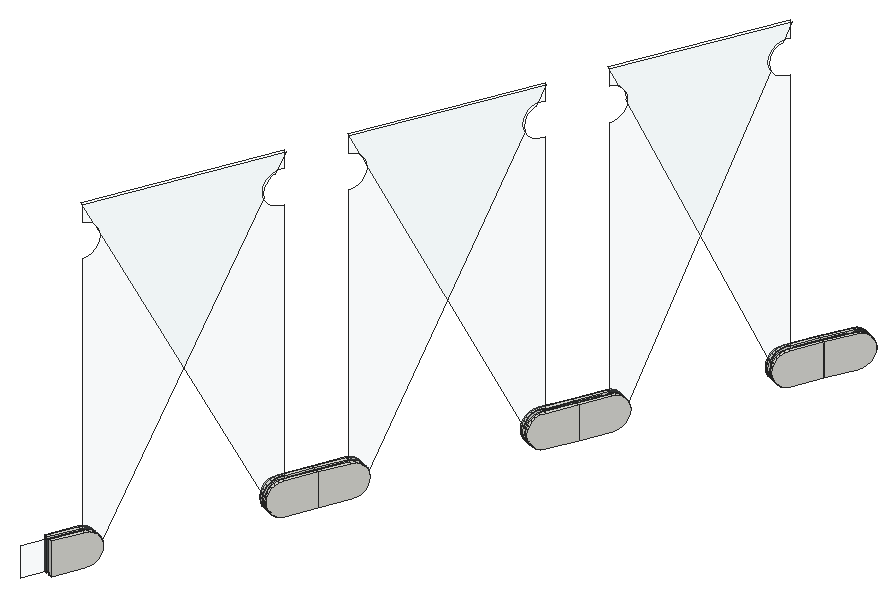
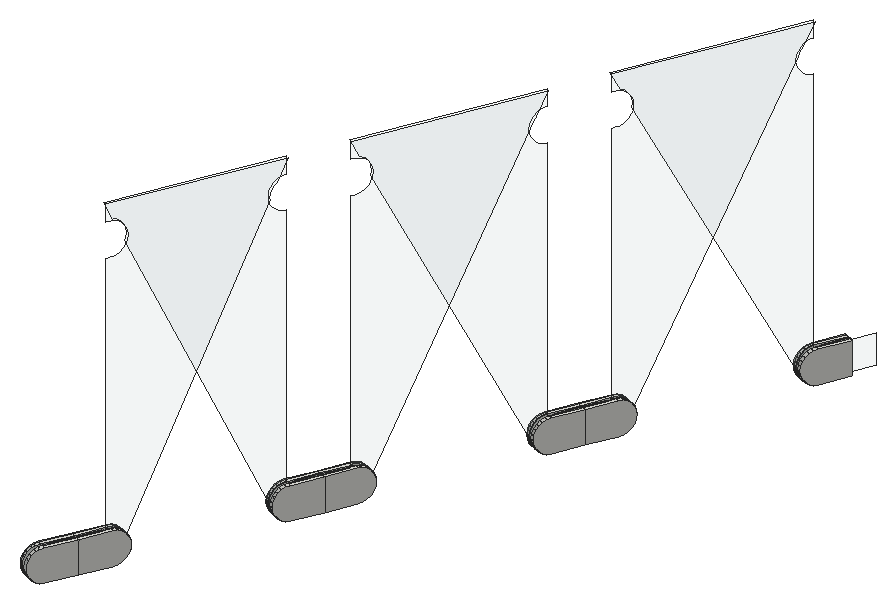
# SketchUp Ruby script. Lengths in inches.
U = 1.inch
M = Sketchup.active_model
def pt(a) = Geom::Point3d.new(a.map { |v| v * U })
def face(e, loops, mat)
  f = e.add_face(loops[0].map { |a| pt(a) })
  loops[1..].each { |l| e.add_face(l.map { |a| pt(a) }).erase! }
  f.material = f.back_material = mat if mat
  f
end
# faces: each face lists its corners as indices into pts; further lists are holes
def faces(e, pts, list, mat = nil) = list.each { |f| face(e, (f[0].is_a?(Array) ? f : [f]).map { |l| l.map { |i| pts[i] } }, mat) }
# xy, xz, yz: faces in a plane at the given z, y or x. An outline is a flat list of corners, or four numbers for a rectangle; further outlines are holes
def ring(l) = l.size == 4 ? [[l[0], l[1]], [l[2], l[1]], [l[2], l[3]], [l[0], l[3]]] : l.each_slice(2).to_a
def flat(e, list, mat, &to3) = list.each { |f| face(e, (f[0].is_a?(Array) ? f : [f]).map { |l| ring(l).map { |u, v| to3.(u, v) } }, mat) }
def xy(e, z, list, mat = nil) = flat(e, list, mat) { |x, y| [x, y, z] }
def xz(e, y, list, mat = nil) = flat(e, list, mat) { |x, z| [x, y, z] }
def yz(e, x, list, mat = nil) = flat(e, list, mat) { |y, z| [x, y, z] }
def lines(e, pts, list) = list.each { |a, b| e.add_line(pt(pts[a]), pt(pts[b])) }
# prism: a flat outline (further loops are holes) pulled along v
def prism(e, loops, v, mat = nil)
  f = face(e, loops, mat); d = Geom::Vector3d.new(v.map { |x| x * U })
  f.pushpull(f.normal.samedirection?(d) ? d.length : -d.length)
end
def box(e, o, s, mat = nil) = prism(e, [[o, [o[0] + s[0], o[1], o[2]], [o[0] + s[0], o[1] + s[1], o[2]], [o[0], o[1] + s[1], o[2]]]], [0, 0, s[2]], mat)
def at(x, y, z, deg = 0) = Geom::Transformation.translation(pt([x, y, z])) * Geom::Transformation.rotation(ORIGIN, Z_AXIS, deg.degrees)
def axes(o, x, y, z) = Geom::Transformation.new([*x, 0, *y, 0, *z, 0, *pt(o).to_a, 1])
def part(name) = M.definitions.add(name)
# library, detail: a bought-in or finely detailed component or shape, given as its bounding box
def library(name, o, s) = part(name).tap { |d| box(d.entities, o, s) }
def detail(e, o, s) = box(e.add_group.entities, o, s)
def put(e, d, t, mat = nil) = e.add_instance(d, t).tap { |i| i.material = mat if mat }
def group(e, t, mat = nil) = e.add_group.tap { |g| g.transformation = t; g.material = mat if mat }.entities
root = M.entities
M.materials.add("Glass_Safety_01").color = [204, 235, 244]
M.materials["Glass_Safety_01"].alpha = 0.1
xy(root,333,[[858.978,571.145,858.726,571.255,859.512,573.06,859.764,572.949],[858.545,571.333,858.292,571.443,859.078,573.248,859.331,573.138],[864.446,583.7,864.194,583.81,864.292,584.037,864.98,585.615,865.232,585.505],[864.013,583.889,863.761,583.999,864.547,585.803,864.799,585.693,864.112,584.115],[865.232,585.505,864.98,585.615,865.766,587.42,866.018,587.309],
  [864.799,585.693,864.547,585.803,865.333,587.608,865.585,587.498],[870.556,597.727,870.303,597.837,870.404,598.069,871.089,599.642,871.341,599.53],[870.122,597.916,869.87,598.026,870.656,599.83,870.908,599.72,870.224,598.148],[871.341,599.53,871.089,599.642,871.342,599.532],[871.342,599.532,871.089,599.642,871.885,601.441,872.137,601.33],
  [870.908,599.72,870.656,599.832,871.453,601.633,871.705,601.521],[876.349,610.851,876.097,610.963,876.207,611.21,876.893,612.761,877.142,612.643],[875.917,611.043,875.665,611.154,876.462,612.954,876.714,612.843,876.027,611.29],[877.142,612.643,876.893,612.761,876.894,612.763,877.146,612.652,877.144,612.647],[877.146,612.652,876.894,612.763,877.734,614.541,877.983,614.423],
  [876.715,612.845,876.466,612.963,877.307,614.743,877.556,614.625]])
xy(root,333.078,[[858.726,571.255,858.545,571.333,859.174,572.777,859.354,572.699],[864.351,584.171,864.17,584.25,864.799,585.693,864.98,585.615],[864.98,585.615,864.799,585.693,865.428,587.137,865.609,587.059],[870.46,598.198,870.28,598.277,870.908,599.72,870.999,599.681,871.089,599.642],[871.089,599.642,870.999,599.681,870.908,599.72,871.546,601.161,871.726,601.081],
  [876.257,611.323,876.077,611.403,876.714,612.843,876.804,612.803,876.893,612.761],[876.893,612.761,876.804,612.803,876.894,612.763,876.893,612.762],[876.894,612.763,876.804,612.803,876.715,612.845,877.388,614.269,877.566,614.185]],"Glass_Safety_01")
xy(root,335.047,[[858.726,571.255,859.354,572.699,859.174,572.777,858.545,571.333],[864.351,584.171,864.98,585.615,864.799,585.693,864.17,584.25],[864.98,585.615,865.609,587.059,865.428,587.137,864.799,585.693],[870.46,598.198,871.089,599.642,870.999,599.681,870.908,599.72,870.28,598.277],[871.089,599.642,871.726,601.081,871.546,601.161,870.908,599.72,870.999,599.681],
  [876.257,611.323,876.893,612.761,876.804,612.803,876.714,612.843,876.077,611.403],[876.893,612.761,876.893,612.762,876.894,612.763,876.804,612.803],[876.894,612.763,877.566,614.185,877.388,614.269,876.715,612.845,876.804,612.803]],"Glass_Safety_01")
xy(root,335.126,[[858.978,571.145,859.764,572.949,859.512,573.06,858.726,571.255],[858.545,571.333,859.331,573.138,859.078,573.248,858.292,571.443],[864.446,583.7,865.232,585.505,864.98,585.615,864.292,584.037,864.194,583.81],[864.013,583.889,864.112,584.115,864.799,585.693,864.547,585.803,863.761,583.999],[865.232,585.505,866.018,587.309,865.766,587.42,864.98,585.615],
  [864.799,585.693,865.585,587.498,865.333,587.608,864.547,585.803],[870.556,597.727,871.341,599.53,871.089,599.642,870.404,598.069,870.303,597.837],[870.122,597.916,870.224,598.148,870.908,599.72,870.656,599.83,869.87,598.026],[871.341,599.53,871.342,599.532,871.089,599.642],[871.342,599.532,872.137,601.33,871.885,601.441,871.089,599.642],
  [870.908,599.72,871.705,601.521,871.453,601.633,870.656,599.832],[876.349,610.851,877.142,612.643,876.893,612.761,876.207,611.21,876.097,610.963],[875.917,611.043,876.027,611.29,876.714,612.843,876.462,612.954,875.665,611.154],[877.142,612.643,877.144,612.647,877.146,612.652,876.894,612.763,876.893,612.761],[877.146,612.652,877.983,614.423,877.734,614.541,876.894,612.763],
  [876.715,612.845,877.556,614.625,877.307,614.743,876.466,612.963]])
p = [[858.726,571.255,333],[858.726,571.255,333.078],[858.726,571.255,335.047],[858.726,571.255,335.126],[858.978,571.145,335.126],[858.978,571.145,333],
  [859.764,572.949,335.126],[859.764,572.949,333],[859.874,573.202,333.036],[859.976,573.437,333.142],[860.064,573.639,333.311],[860.132,573.793,333.531],
  [860.174,573.891,333.787],[860.189,573.924,334.0625],[860.174,573.891,334.338],[860.132,573.793,334.594],[860.064,573.639,334.814],[859.976,573.437,334.983],
  [859.874,573.202,335.089],[858.545,571.333,333.078],[858.545,571.333,333],[858.292,571.443,333],[858.292,571.443,335.126],[858.545,571.333,335.126],
  [858.545,571.333,335.047],[859.331,573.138,333],[859.331,573.138,335.126],[859.174,572.777,335.047],[859.174,572.777,333.078],[859.512,573.06,335.126],
  [859.512,573.06,333],[859.354,572.699,333.078],[859.354,572.699,335.047],[859.078,573.248,335.126],[859.188,573.5,335.089],[859.291,573.735,334.983],
  [859.379,573.9375,334.814],[859.446,574.092,334.594],[859.488,574.19,334.338],[859.503,574.223,334.0625],[859.488,574.19,333.787],[859.446,574.092,333.531],
  [859.379,573.9375,333.311],[859.291,573.735,333.142],[859.188,573.5,333.036],[859.078,573.248,333],[859.621,573.312,333.036],[859.441,573.39,333.036],
  [859.441,573.39,335.089],[859.543,573.625,334.983],[859.631,573.827,334.814],[859.699,573.982,334.594],[859.741,574.08,334.338],[859.756,574.113,334.0625],
  [859.741,574.08,333.787],[859.699,573.982,333.531],[859.631,573.827,333.311],[859.543,573.625,333.142],[859.925,574.009,333.853],[859.81,573.744,333.307],
  [859.724,573.547,333.142],[859.621,573.312,335.089],[859.724,573.547,334.983],[859.812,573.749,334.814],[859.879,573.904,334.594],[859.922,574.001,334.338],
  [859.936,574.034,334.0625],[865.232,585.505,335.126],[864.446,583.7,335.126],[864.337,583.448,335.089],[864.234,583.213,334.983],[864.146,583.011,334.814],
  [864.079,582.856,334.594],[864.036,582.759,334.338],[864.022,582.725,334.0625],[864.036,582.759,333.787],[864.079,582.856,333.531],[864.146,583.011,333.311],
  [864.234,583.213,333.142],[864.337,583.448,333.036],[864.446,583.7,333],[865.232,585.505,333],[864.194,583.81,335.126],[864.292,584.037,335.126],
  [864.292,584.037,333],[864.194,583.81,333],[864.084,583.558,333.036],[863.981,583.323,333.142],[863.894,583.121,333.311],[863.826,582.966,333.531],
  [863.784,582.869,333.787],[863.769,582.835,334.0625],[863.784,582.869,334.338],[863.826,582.966,334.594],[863.894,583.121,334.814],[863.981,583.323,334.983],
  [864.084,583.558,335.089],[863.602,582.944,334.311],[863.862,583.542,333.078],[863.903,583.636,333.036],[864.013,583.889,333],[864.112,584.115,333],
  [864.112,584.115,335.126],[864.013,583.889,335.126],[863.903,583.636,335.089],[863.801,583.401,334.983],[863.713,583.199,334.814],[863.646,583.045,334.594],
  [863.603,582.947,334.338],[863.761,583.999,335.126],[864.547,585.803,335.126],[864.547,585.803,333],[863.761,583.999,333],[863.651,583.746,333.036],
  [863.548,583.511,333.142],[863.46,583.31,333.311],[863.393,583.155,333.531],[863.351,583.057,333.787],[863.336,583.024,334.0625],[863.351,583.057,334.338],
  [863.393,583.155,334.594],[863.46,583.31,334.814],[863.548,583.511,334.983],[863.651,583.746,335.089],[863.801,583.401,333.142],[864.98,585.615,333],
  [864.98,585.615,335.126],[864.98,585.615,335.047],[864.351,584.171,335.047],[864.351,584.171,333.078],[864.98,585.615,333.078],[864.799,585.693,335.126],
  [864.799,585.693,333],[864.799,585.693,333.078],[864.17,584.25,333.078],[864.17,584.25,335.047],[864.799,585.693,335.047],[866.018,587.309,335.126],
  [866.018,587.309,333],[866.128,587.562,333.036],[866.231,587.797,333.142],[866.319,587.999,333.311],[866.386,588.153,333.531],[866.428,588.251,333.787],
  [866.443,588.284,334.0625],[866.428,588.251,334.338],[866.386,588.153,334.594],[866.319,587.999,334.814],[866.231,587.797,334.983],[866.128,587.562,335.089],
  [865.766,587.42,335.126],[865.766,587.42,333],[865.609,587.059,333.078],[865.609,587.059,335.047],[865.585,587.498,333],[865.585,587.498,335.126],
  [865.428,587.137,335.047],[865.428,587.137,333.078],[865.333,587.608,335.126],[865.442,587.86,335.089],[865.545,588.095,334.983],[865.633,588.297,334.814],
  [865.7,588.452,334.594],[865.743,588.55,334.338],[865.757,588.583,334.0625],[865.743,588.55,333.787],[865.7,588.452,333.531],[865.633,588.297,333.311],
  [865.545,588.095,333.142],[865.442,587.86,333.036],[865.333,587.608,333],[865.876,587.672,333.036],[866.183,588.379,333.934],[866.049,588.07,333.279],
  [865.978,587.907,333.142],[865.876,587.672,335.089],[865.978,587.907,334.983],[866.066,588.109,334.814],[866.133,588.264,334.594],[866.176,588.361,334.338],
  [866.19,588.394,334.0625],[865.695,587.75,333.036],[865.695,587.75,335.089],[865.798,587.985,334.983],[865.885,588.187,334.814],[865.953,588.342,334.594],
  [865.995,588.439,334.338],[866.01,588.473,334.0625],[865.995,588.439,333.787],[865.953,588.342,333.531],[865.885,588.187,333.311],[865.798,587.985,333.142],
  [870.556,597.727,333],[871.341,599.53,333],[871.341,599.53,335.126],[870.556,597.727,335.126],[870.446,597.475,335.089],[870.343,597.24,334.983],
  [870.255,597.038,334.814],[870.188,596.883,334.594],[870.146,596.786,334.338],[870.131,596.752,334.0625],[870.146,596.786,333.787],[870.188,596.883,333.531],
  [870.255,597.038,333.311],[870.343,597.24,333.142],[870.446,597.475,333.036],[870.303,597.837,335.126],[870.404,598.069,335.126],[870.404,598.069,333],
  [870.303,597.837,333],[870.193,597.585,333.036],[870.091,597.35,333.142],[870.003,597.148,333.311],[869.935,596.993,333.531],[869.893,596.896,333.787],
  [869.878,596.862,334.0625],[869.893,596.896,334.338],[869.935,596.993,334.594],[870.003,597.148,334.814],[870.091,597.35,334.983],[870.193,597.585,335.089],
  [869.717,596.985,334.366],[869.984,597.598,333.065],[870.013,597.663,333.036],[870.122,597.916,333],[870.224,598.148,333],[870.224,598.148,335.126],
  [870.122,597.916,335.126],[870.013,597.663,335.089],[869.91,597.428,334.983],[869.822,597.226,334.814],[869.755,597.072,334.594],[869.87,598.026,335.126],
  [870.656,599.83,335.126],[870.656,599.83,333],[869.87,598.026,333],[869.76,597.773,333.036],[869.658,597.538,333.142],[869.57,597.337,333.311],
  [869.502,597.182,333.531],[869.46,597.084,333.787],[869.445,597.051,334.0625],[869.46,597.084,334.338],[869.502,597.182,334.594],[869.57,597.337,334.814],
  [869.658,597.538,334.983],[869.76,597.773,335.089],[869.91,597.428,333.142],[870.908,599.72,335.126],[870.908,599.72,333],[870.908,599.72,333.078],
  [870.28,598.277,333.078],[870.28,598.277,335.047],[870.908,599.72,335.047],[871.089,599.642,333],[871.089,599.642,335.126],[871.089,599.642,335.047],
  [870.46,598.198,335.047],[870.46,598.198,333.078],[871.089,599.642,333.078],[871.342,599.532,335.126],[871.342,599.532,333],[872.137,601.33,335.126],
  [872.137,601.33,333],[872.248,601.582,333.036],[872.352,601.816,333.142],[872.441,602.017,333.311],[872.51,602.172,333.531],[872.553,602.269,333.787],
  [872.567,602.302,334.0625],[872.553,602.269,334.338],[872.51,602.172,334.594],[872.441,602.017,334.814],[872.352,601.816,334.983],[872.248,601.582,335.089],
  [871.885,601.441,335.126],[871.885,601.441,333],[871.726,601.081,333.078],[871.726,601.081,335.047],[870.656,599.832,335.126],[870.656,599.832,333],
  [871.705,601.521,333],[871.705,601.521,335.126],[871.546,601.161,335.047],[871.546,601.161,333.078],[871.453,601.633,335.126],[871.564,601.884,335.089],
  [871.668,602.119,334.983],[871.757,602.32,334.814],[871.825,602.474,334.594],[871.868,602.572,334.338],[871.883,602.605,334.0625],[871.868,602.572,333.787],
  [871.825,602.474,333.531],[871.757,602.32,333.311],[871.668,602.119,333.142],[871.564,601.884,333.036],[871.453,601.633,333],[871.996,601.693,333.036],
  [872.312,602.406,334.129],[872.136,602.008,333.21],[872.1,601.927,333.142],[871.996,601.693,335.089],[872.1,601.927,334.983],[872.189,602.129,334.814],
  [872.258,602.283,334.594],[872.3,602.38,334.338],[871.816,601.773,333.036],[871.816,601.773,335.089],[871.92,602.007,334.983],[872.009,602.208,334.814],
  [872.077,602.363,334.594],[872.12,602.46,334.338],[872.135,602.493,334.0625],[872.12,602.46,333.787],[872.077,602.363,333.531],[872.009,602.208,333.311],
  [871.92,602.007,333.142],[876.349,610.851,333],[877.142,612.643,333],[877.142,612.643,335.126],[876.349,610.851,335.126],[876.238,610.6,335.089],
  [876.134,610.365,334.983],[876.045,610.164,334.814],[875.977,610.01,334.594],[875.934,609.912,334.338],[875.919,609.879,334.0625],[875.934,609.912,333.787],
  [875.977,610.01,333.531],[876.045,610.164,333.311],[876.134,610.365,333.142],[876.238,610.6,333.036],[876.207,611.21,333],[876.207,611.21,335.126],
  [876.097,610.963,335.126],[875.986,610.711,335.089],[875.882,610.477,334.983],[875.793,610.276,334.814],[875.725,610.121,334.594],[875.682,610.024,334.338],
  [875.667,609.991,334.0625],[875.682,610.024,333.787],[875.725,610.121,333.531],[875.793,610.276,333.311],[875.882,610.477,333.142],[875.986,610.711,333.036],
  [876.097,610.963,333],[876.893,612.761,335.126],[876.893,612.761,335.047],[876.893,612.761,333.078],[876.893,612.761,333],[875.529,610.165,334.5],
  [875.502,610.104,334.338],[875.487,610.07,334.0625],[875.502,610.104,333.787],[875.545,610.201,333.531],[875.613,610.355,333.311],[875.702,610.557,333.142],
  [875.806,610.791,333.036],[875.809,610.798,333.035],[875.665,611.154,335.126],[876.462,612.954,335.126],[876.462,612.954,333],[875.665,611.154,333],
  [875.554,610.902,333.036],[875.45,610.668,333.142],[875.361,610.467,333.311],[875.293,610.312,333.531],[875.25,610.215,333.787],[875.235,610.182,334.0625],
  [875.25,610.215,334.338],[875.293,610.312,334.594],[875.361,610.467,334.814],[875.45,610.668,334.983],[875.554,610.902,335.089],[875.917,611.043,333],
  [876.027,611.29,333],[876.027,611.29,335.126],[875.917,611.043,335.126],[875.806,610.791,335.089],[875.702,610.557,334.983],[875.613,610.355,334.814],
  [875.545,610.201,334.594],[876.714,612.843,335.126],[876.714,612.843,333],[876.714,612.843,333.078],[876.077,611.403,333.078],[876.077,611.403,335.047],
  [876.714,612.843,335.047],[877.144,612.647,335.126],[877.144,612.647,333],[877.146,612.652,333],[877.146,612.652,335.126],[877.983,614.423,333],
  [878.101,614.672,333.036],[878.21,614.903,333.142],[878.304,615.103,333.311],[878.376,615.255,333.531],[878.422,615.351,333.787],[878.437,615.384,334.0625],
  [878.422,615.351,334.338],[878.376,615.255,334.594],[878.304,615.103,334.814],[878.21,614.903,334.983],[878.101,614.672,335.089],[877.983,614.423,335.126],
  [876.894,612.763,333],[876.894,612.763,333.078],[876.894,612.763,335.047],[876.894,612.763,335.126],[876.715,612.845,333],[876.715,612.845,333.078],
  [876.715,612.845,335.047],[876.715,612.845,335.126],[876.466,612.963,335.126],[876.466,612.963,333],[877.556,614.625,333],[877.556,614.625,335.126],
  [877.388,614.269,335.047],[877.388,614.269,333.078],[877.734,614.541,335.126],[877.851,614.789,335.089],[877.961,615.021,334.983],[878.055,615.22,334.814],
  [878.127,615.373,334.594],[878.173,615.469,334.338],[878.188,615.502,334.0625],[878.181,615.487,333.943],[878.173,615.469,333.787],[878.127,615.373,333.531],
  [878.055,615.22,333.311],[878.035,615.179,333.276],[877.961,615.021,333.142],[877.851,614.789,333.036],[877.734,614.541,333],[877.307,614.743,335.126],
  [877.424,614.991,335.089],[877.534,615.223,334.983],[877.628,615.422,334.814],[877.7,615.575,334.594],[877.745,615.671,334.338],[877.761,615.704,334.0625],
  [877.745,615.671,333.787],[877.7,615.575,333.531],[877.628,615.422,333.311],[877.534,615.223,333.142],[877.424,614.991,333.036],[877.307,614.743,333],
  [877.673,614.874,333.036],[877.673,614.874,335.089],[877.783,615.105,334.983],[877.877,615.304,334.814],[877.949,615.457,334.594],[877.995,615.553,334.338],
  [878.01,615.586,334.0625],[877.995,615.553,333.787],[877.949,615.457,333.531],[877.877,615.304,333.311],[877.783,615.105,333.142],[857.916,569.89,333.078],
  [857.916,569.89,335.047],[859.812,573.749,333.311],[863.589,582.914,334.0625],[863.603,582.947,333.787],[863.646,583.045,333.531],[863.713,583.199,333.311],
  [866.066,588.109,333.311],[869.712,596.974,334.338],[869.698,596.941,334.0625],[869.712,596.974,333.787],[869.755,597.072,333.531],[869.822,597.226,333.311],
  [870.999,599.681,333.078],[870.999,599.681,335.047],[872.189,602.129,333.311],[876.257,611.323,333.078],[876.257,611.323,335.047],[876.804,612.803,335.047],
  [876.804,612.803,333.078],[876.893,612.762,333.078],[876.893,612.762,335.047],[877.566,614.185,335.047],[877.566,614.185,333.078],[872.258,602.283,333.531],
  [872.3,602.38,333.787],[872.315,602.414,334.0625],[859.879,573.904,333.531],[859.922,574.001,333.787],[866.133,588.264,333.531],[866.176,588.361,333.787],
  [859.512,573.06,351.283],[863.782,582.865,352.098],[863.769,582.835,352.346],[863.784,582.869,352.621],[863.826,582.966,352.877],[863.894,583.121,353.098],
  [863.981,583.323,353.267],[864.043,583.463,353.33],[864.292,584.037,354.511],[859.512,573.06,354.511],[859.512,573.06,353.409],[859.621,573.312,353.373],
  [859.724,573.547,353.267],[859.812,573.749,353.098],[859.879,573.904,352.877],[859.922,574.001,352.621],[859.936,574.034,352.346],[859.922,574.001,352.071],
  [859.879,573.904,351.815],[859.812,573.749,351.594],[859.724,573.547,351.425],[859.621,573.312,351.319],[865.766,587.42,351.283],[869.898,596.906,352.042],
  [869.893,596.896,352.071],[869.878,596.862,352.346],[869.893,596.896,352.621],[869.935,596.993,352.877],[870.003,597.148,353.098],[870.091,597.35,353.267],
  [870.164,597.519,353.343],[870.404,598.069,354.511],[865.766,587.42,354.511],[865.766,587.42,353.409],[865.876,587.672,353.373],[865.978,587.907,353.267],
  [866.066,588.109,353.098],[866.133,588.264,352.877],[866.176,588.361,352.621],[866.19,588.394,352.346],[866.176,588.361,352.071],[866.133,588.264,351.815],
  [866.066,588.109,351.594],[865.978,587.907,351.425],[865.876,587.672,351.319],[875.709,610.086,351.908],[875.682,610.024,352.071],[875.667,609.991,352.346],
  [875.682,610.024,352.621],[875.725,610.121,352.877],[875.793,610.276,353.098],[875.882,610.477,353.267],[875.986,610.711,353.373],[875.989,610.719,353.374],
  [876.207,611.21,354.511],[871.885,601.441,354.511],[871.885,601.441,353.409],[871.996,601.693,353.373],[872.1,601.927,353.267],[872.189,602.129,353.098],
  [872.258,602.283,352.877],[872.3,602.38,352.621],[872.315,602.414,352.346],[872.3,602.38,352.071],[872.258,602.283,351.815],[872.189,602.129,351.594],
  [872.1,601.927,351.425],[871.996,601.693,351.319],[871.885,601.441,351.283],[859.745,574.087,352.556],[859.741,574.08,352.621],[859.699,573.982,352.877],
  [859.631,573.827,353.098],[859.629,573.822,353.102],[859.331,573.138,354.511],[864.112,584.115,354.511],[864.112,584.115,353.409],[864.013,583.889,353.409],
  [863.903,583.636,353.373],[863.801,583.401,353.267],[863.713,583.199,353.098],[863.646,583.045,352.877],[863.603,582.947,352.621],[863.589,582.914,352.346],
  [863.603,582.947,352.071],[863.646,583.045,351.815],[863.713,583.199,351.594],[863.801,583.401,351.425],[863.903,583.636,351.319],[864.013,583.889,351.283],
  [864.112,584.115,351.283],[866.003,588.457,352.475],[865.995,588.439,352.621],[865.953,588.342,352.877],[865.885,588.187,353.098],[865.869,588.149,353.13],
  [865.585,587.498,354.511],[870.224,598.148,354.511],[870.224,598.148,353.409],[870.122,597.916,353.409],[870.013,597.663,353.373],[869.91,597.428,353.267],
  [869.822,597.226,353.098],[869.755,597.072,352.877],[869.712,596.974,352.621],[869.698,596.941,352.346],[869.712,596.974,352.071],[869.755,597.072,351.815],
  [869.822,597.226,351.594],[869.91,597.428,351.425],[870.013,597.663,351.319],[870.122,597.916,351.283],[870.224,598.148,351.283],[872.132,602.485,352.279],
  [872.135,602.493,352.346],[872.12,602.46,352.621],[872.077,602.363,352.877],[872.009,602.208,353.098],[871.956,602.088,353.199],[871.705,601.521,354.511],
  [876.027,611.29,354.511],[876.027,611.29,353.409],[875.917,611.043,353.409],[875.806,610.791,353.373],[875.702,610.557,353.267],[875.613,610.355,353.098],
  [875.545,610.201,352.877],[875.502,610.104,352.621],[875.487,610.07,352.346],[875.502,610.104,352.071],[875.545,610.201,351.814],[875.613,610.355,351.594],
  [875.702,610.557,351.425],[875.806,610.791,351.319],[875.917,611.043,351.283],[876.027,611.29,351.283]]
faces(root,p,[[0,1,2,3,4,5],[6,4,5,7,8,9,10,11,12,13,14,15,16,17,18],[19,20,21,22,23,24],[20,25,26,23,24,27,28,19],[3,29,30,0,1,31,32,2],[22,33,34,35,36,37,38,39,40,41,42,43,44,45,21],[30,46,8,7],[47,25,45,44],
  [46,60,9,8],[57,47,44,43],[67,68,69,70,71,72,73,74,75,76,77,78,79,80,81],[82,83,84,85,86,87,88,89,90,91,92,93,94,95,96],[109,110,111,112,113,114,115,116,117,118,119,120,121,122,123],[87,86,79,78],[98,124,114,113,99],[86,85,80,79],
  [100,99,113,112],[125,84,83,126,127,128,129,130],[131,102,101,132,133,134,135,136],[125,130,127,126,67,81],[137,67,81,138,139,140,141,142,143,144,145,146,147,148,149],[126,150,151,125,130,152,153,127],[133,132,111,110,131,136],[132,154,155,131,136,156,157,133],
  [110,158,159,160,161,162,163,164,165,166,167,168,169,170,111],[151,171,139,138],[181,154,170,169],[171,174,140,139],[191,181,169,168],[192,193,194,195,196,197,198,199,200,201,202,203,204,205,206],[207,208,209,210,211,212,213,214,215,216,217,218,219,220,221],[233,234,235,236,237,238,239,240,241,242,243,244,245,246,247],
  [212,211,206,205],[223,248,238,237,224],[211,210,192,206],[225,224,237,236],[249,227,226,250,251,252,253,254],[255,209,208,256,257,258,259,260],[260,255,193,194,256,257],[255,260,257,256,261,262],
  [193,262,261,194],[263,261,262,264,265,266,267,268,269,270,271,272,273,274,275],[256,276,277,255,260,278,279,257],[251,250,235,234,249,254],[250,251,254,249,280,281],[250,282,283,249,254,284,285,251],[280,286,287,288,289,290,291,292,293,294,295,296,297,298,281],[277,299,265,264],
  [308,282,298,297],[299,302,266,265],[318,308,297,296],[319,320,321,322,323,324,325,326,327,328,329,330,331,332,333],[335,349,350,351,352,334,348,347,346,345,344,343,342,341,340,339,338,337,336],[353,354,355,356,357,358,359,360,361],[362,363,364,365,366,367,368,369,370,371,372,373,374,375,376],[346,347,333,332],
  [360,359,367,366],[347,348,319,333],[361,360,366,365,377],[385,379,378,386,387,388,389,390],[351,352,320,321,349,350],[391,321,320,392,393,394],[391,321,320,392,393,395,396,397,398,399,400,401,402,403,404,405,406,407,394],[408,409,410,411,394,393],
  [387,386,364,363,385,390],[412,413,414,415,416,417],[412,418,419,415,414,420,421,413],[408,352,351,350,349,411,410,409],[349,411,422,423,424,425,426,427,428,429,430,431,432,433,434,435,436,408,352,351,350],[416,437,438,439,440,441,442,443,444,445,446,447,448,449,417],[436,435,396,395],[450,418,449,448],
  [435,434,397,396],[460,450,448,447],[59,463,10,9,60],[56,57,43,42],[97,464,465,466,467,124,98],[88,87,78,77],[124,467,115,114],[173,468,141,140,174],
  [190,191,168,167],[222,469,470,471,472,473,248,223],[213,212,205,204],[248,473,239,238],[301,476,267,266,302],[317,318,296,295],[345,346,332,331],[359,358,368,367],
  [433,432,398,397,434],[459,460,447,446],[463,488,11,10],[55,56,42,41],[89,88,77,76],[467,466,116,115],[468,490,142,141],[189,190,167,166],
  [214,213,204,203],[473,472,240,239],[476,485,268,267],[316,317,295,294],[344,345,331,330],[358,357,369,368],[432,431,399,398],[458,459,446,445],
  [488,489,12,11],[54,55,41,40],[90,89,76,75],[466,465,117,116],[490,491,143,142],[188,189,166,165],[215,214,203,202],[472,471,241,240],
  [485,486,269,268],[315,316,294,293],[343,344,330,329],[357,356,370,369],[431,430,400,399],[457,458,445,444],[58,66,13,12,489],[53,54,40,39],
  [91,90,75,74],[465,464,118,117],[172,180,144,143,491],[187,188,165,164],[216,215,202,201],[471,470,242,241],[486,487,270,269],[314,315,293,292],
  [342,343,329,328],[356,355,371,370],[429,428,401,400,430],[66,65,14,13],[52,53,39,38],[92,91,74,73],[97,108,119,118,464],[180,179,145,144],
  [186,187,164,163],[217,216,201,200],[470,469,243,242],[300,307,271,270,487],[313,314,292,291],[341,342,328,327],[355,354,372,371],[428,427,402,401],
  [65,64,15,14],[51,52,38,37],[93,92,73,72],[108,107,120,119],[179,178,146,145],[185,186,163,162],[218,217,200,199],[222,232,244,243,469],
  [307,306,272,271],[312,313,291,290],[340,341,327,326],[353,384,373,372,354],[427,426,403,402],[64,63,16,15],[50,51,37,36],[94,93,72,71],
  [107,106,121,120],[178,177,147,146],[184,185,162,161],[219,218,199,198],[232,231,245,244],[306,305,273,272],[311,312,290,289],[339,340,326,325],
  [384,383,374,373],[426,425,404,403],[453,454,441,440],[63,62,17,16],[49,50,36,35],[95,94,71,70],[106,105,122,121],[177,176,148,147],
  [183,184,161,160],[220,219,198,197],[231,230,246,245],[305,304,274,273],[310,311,289,288],[338,339,325,324],[383,382,375,374],[425,424,405,404],
  [452,453,440,439],[62,61,18,17],[48,49,35,34],[96,95,70,69],[105,104,123,122],[176,175,149,148],[182,183,160,159],[221,220,197,196],
  [230,229,247,246],[304,303,275,274],[309,310,288,287],[337,338,324,323],[382,381,376,375],[424,423,406,405],[451,452,439,438],[61,29,6,18],
  [26,48,34,33],[82,96,69,68],[104,103,109,123],[175,150,137,149],[155,182,159,158],[207,221,196,195],[229,228,233,247],[303,276,263,275],
  [283,309,287,286],[336,337,323,322],[381,380,362,376],[423,422,407,406],[419,451,438,437]])
faces(root,p,[[25,26,48,49,50,51,52,53,54,55,56,57,47],[58,59,60,46,30,29,61,62,63,64,65,66],[97,98,99,100,101,102,103,104,105,106,107,108],[172,173,174,171,151,150,175,176,177,178,179,180],[154,155,182,183,184,185,186,187,188,189,190,191,181],[222,223,224,225,226,227,228,229,230,231,232],[300,301,302,299,277,276,303,304,305,306,307],[282,283,309,310,311,312,313,314,315,316,317,318,308],
  [334,335,336,337,338,339,340,341,342,343,344,345,346,347,348],[353,361,377,378,379,380,381,382,383,384],[433,429,428,427,426,425,424,423,422,436,435,434],[418,419,451,452,453,454,455,456,457,458,459,460,450],[461,19,24,462],[24,2,1,19],[19,28,27,24],[31,1,2,32],
  [32,31,28,27],[129,128,135,134],[134,133,136,135],[130,129,128,127],[136,127,130,133],[152,130,127,153],[133,157,156,136],[153,152,157,156],
  [259,258,253,252],[260,259,258,257],[252,251,254,253],[260,474,475,257],[278,260,257,279],[254,475,474,251],[251,285,284,254],[284,279,278,285],
  [477,478,389,388],[477,351,350,478],[388,387,390,389],[390,479,480,387],[480,479,414,413],[413,421,420,414],[479,480,351,350],[409,480,479,410],
  [481,409,410,482,350,351],[483,410,409,484],[420,483,484,421],[300,301,476,485,486,487],[58,59,463,488,489],[172,173,468,490,491],[429,433,432,431,430],[492,29,61,62,63,64,65,66,58,493,494,495,496,497,498,499,500,501,502,503,504,505,506,507,508,509,510,511,512,513],
  [514,150,175,176,177,178,179,180,172,515,516,517,518,519,520,521,522,523,524,525,526,527,528,529,530,531,532,533,534,535,536],[300,537,538,539,540,541,542,543,544,545,546,547,548,549,550,551,552,553,554,555,556,557,558,559,560,276,303,304,305,306,307],[97,561,562,563,564,565,566,567,568,569,570,571,572,573,574,575,576,577,578,579,580,581,582,102,103,104,105,106,107,108],[222,583,584,585,586,587,588,589,590,591,592,593,594,595,596,597,598,599,600,601,602,603,604,227,228,229,230,231,232],[353,605,606,607,608,609,610,611,612,613,614,615,616,617,618,619,620,621,622,623,624,625,626,627,379,380,381,382,383,384]],"Glass_Safety_01")
